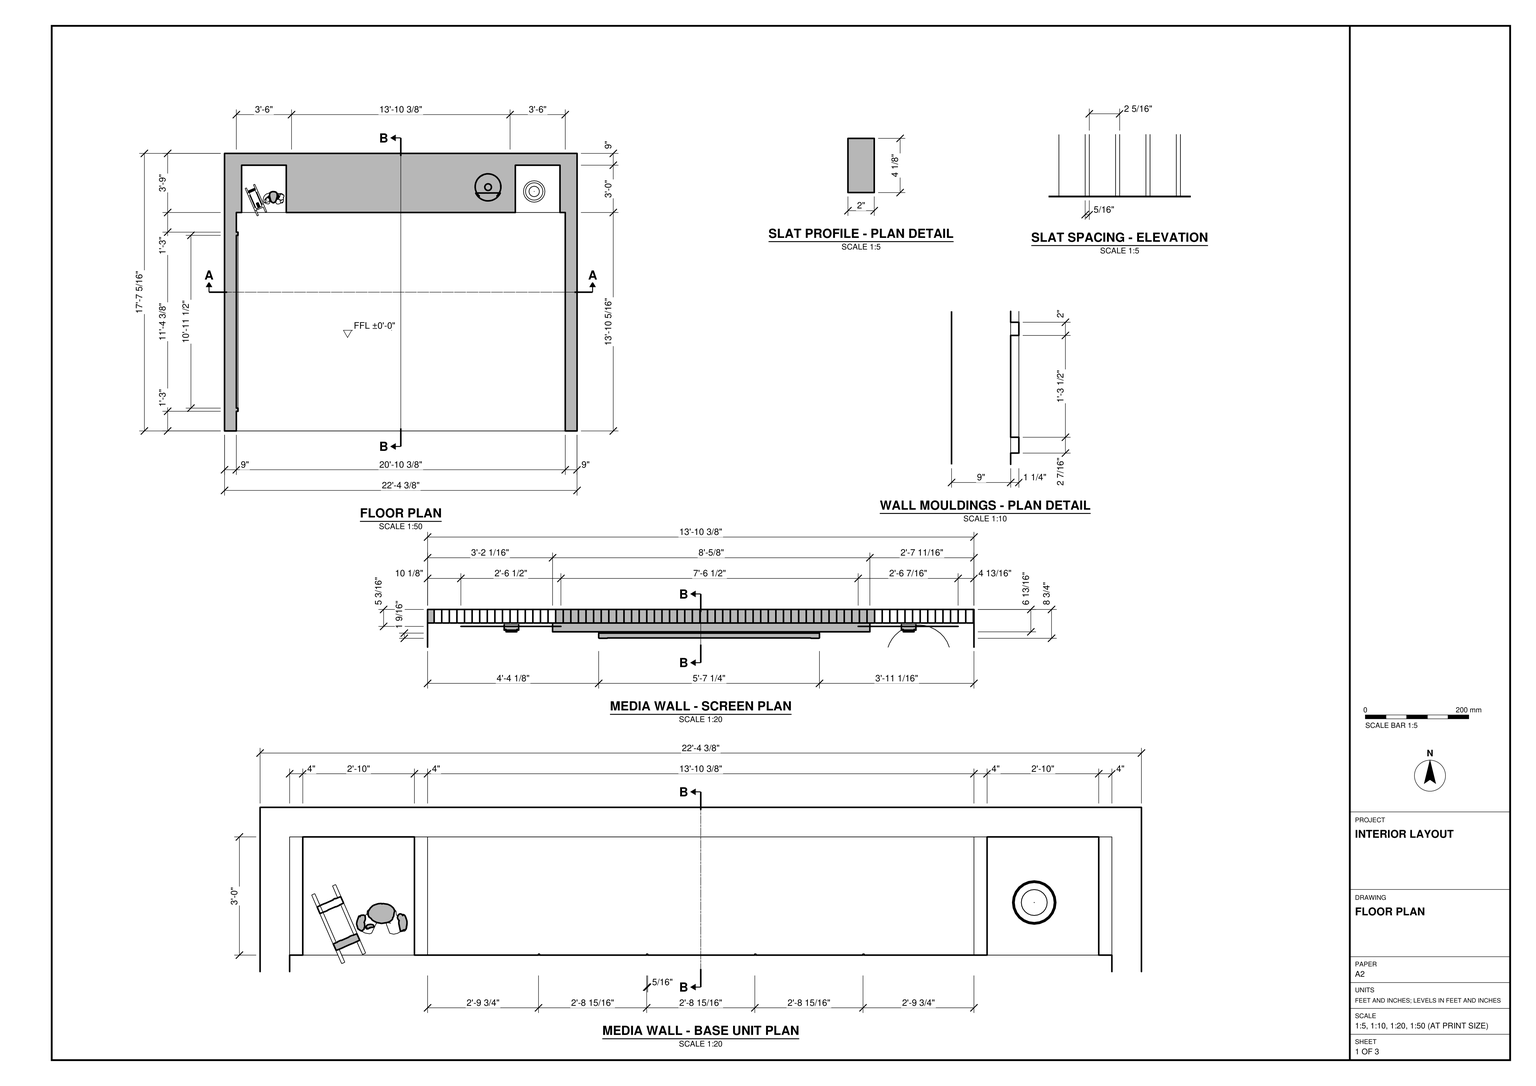
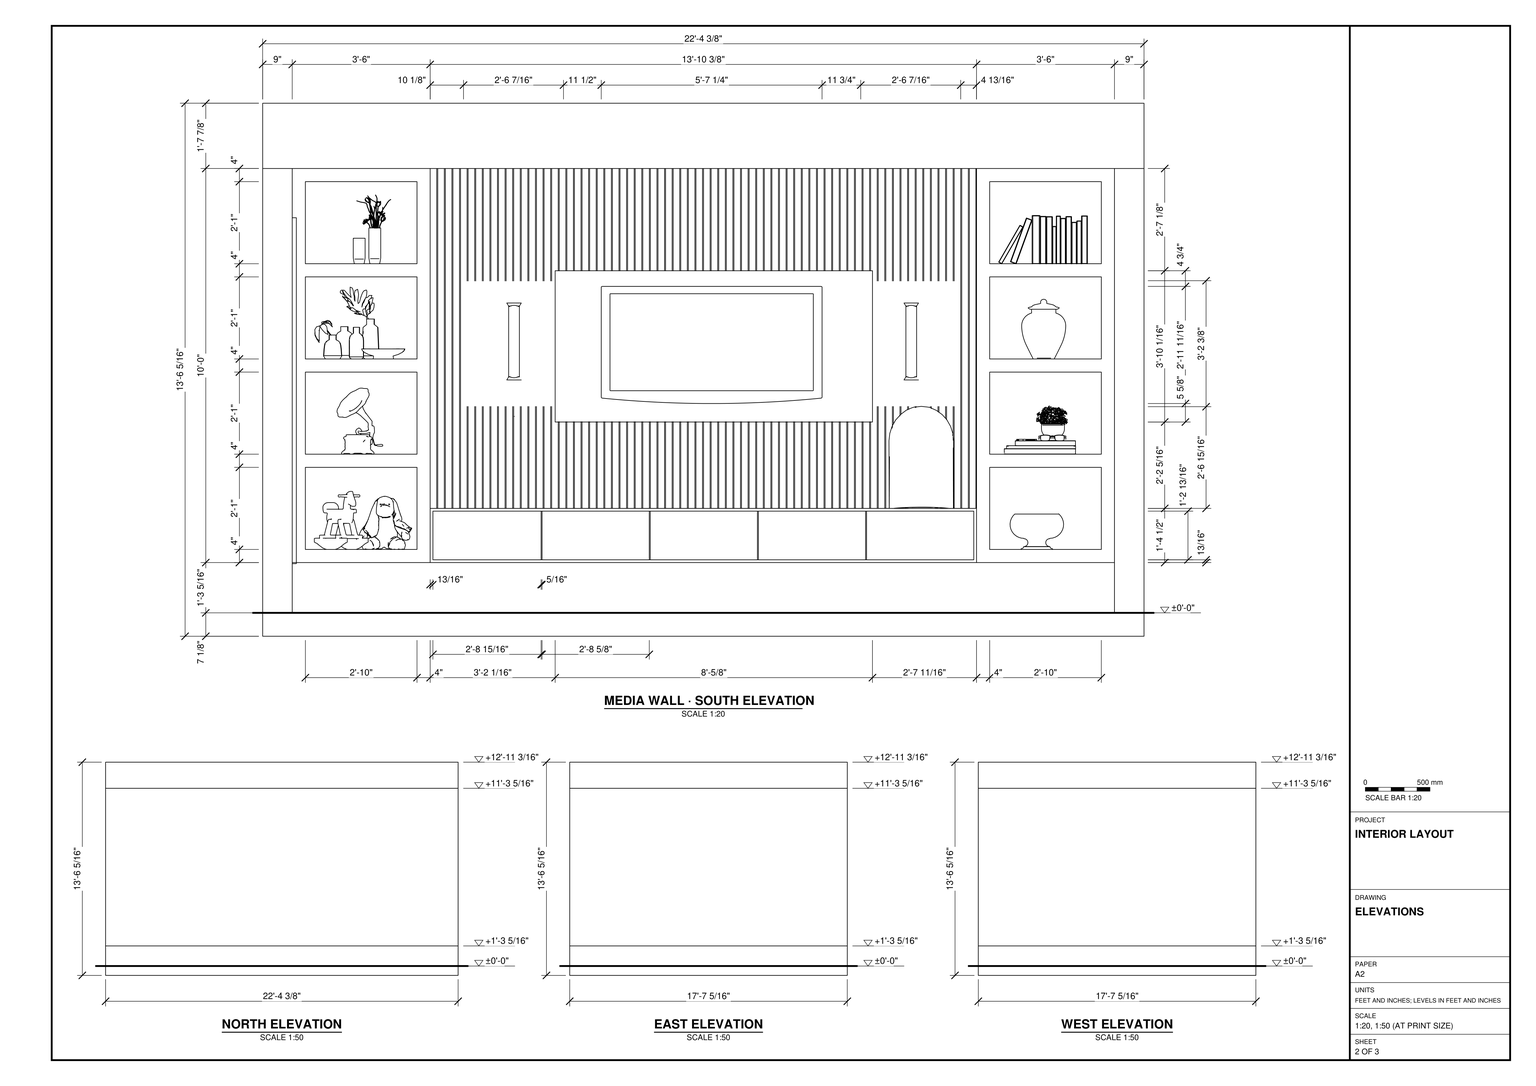
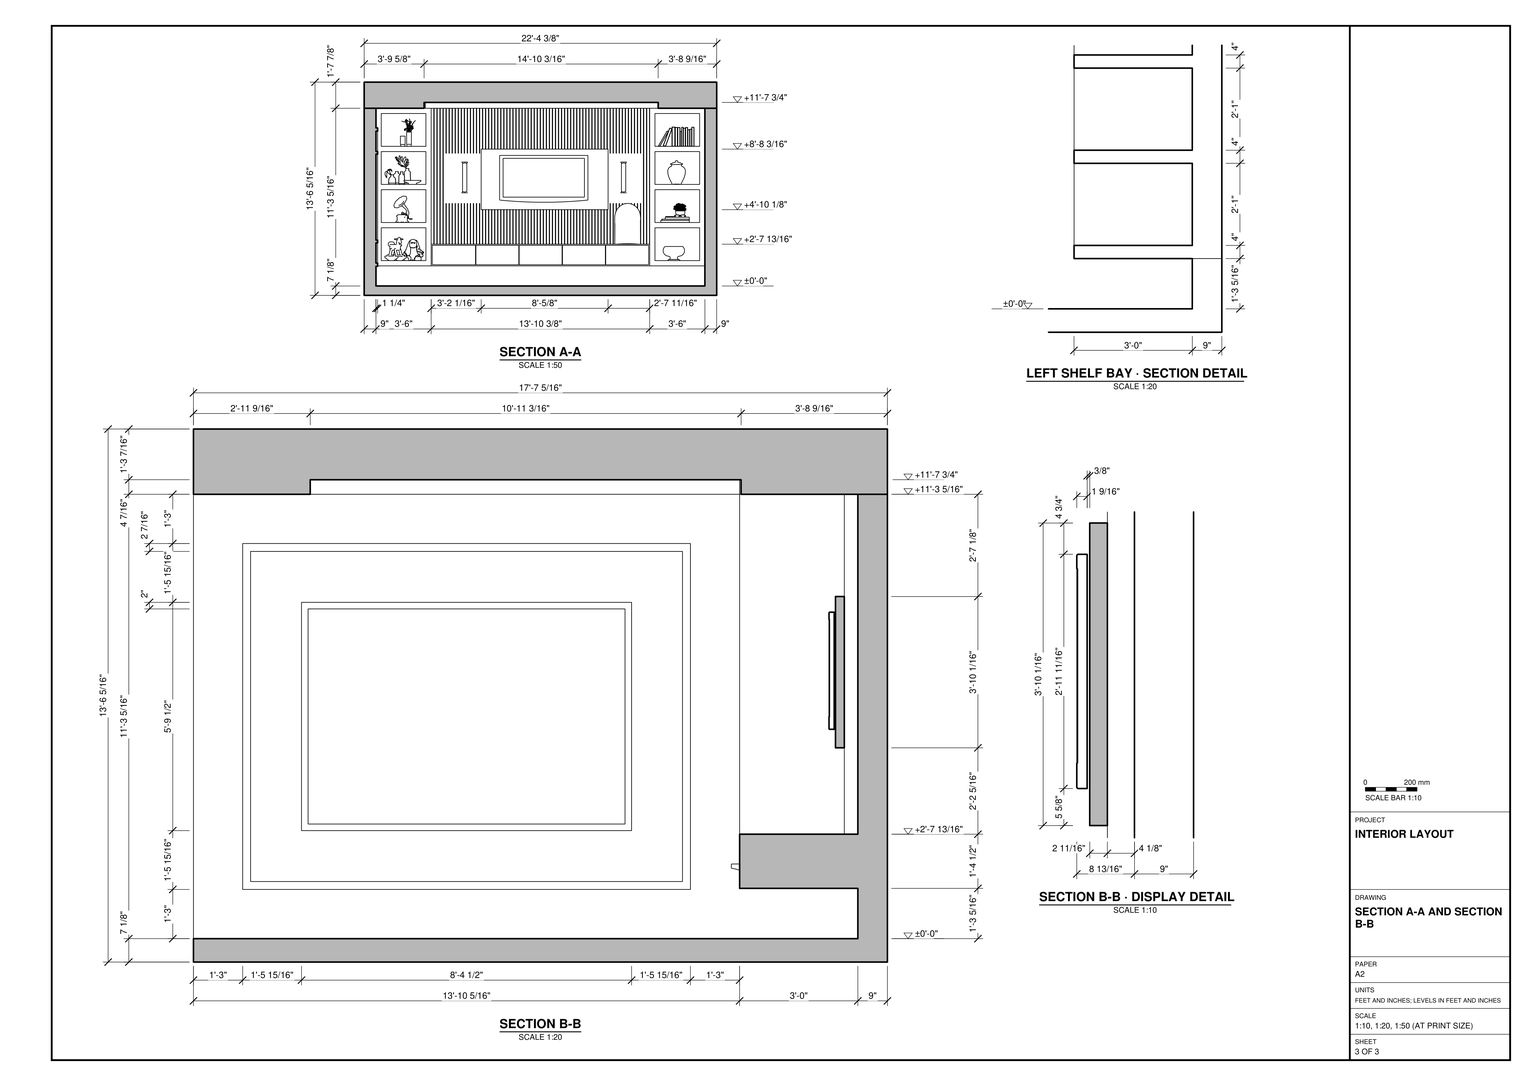
Build the room in SketchUp from task_files/diagram_01.pdf. Work in feet and inches. The overall dimensions are 22'-4 3/8" wide by 17'-7 5/16" deep by 13'-6 5/16" high, with the finished floor at ±0'-0". Follow the plan for the three-sided enclosure, leaving the front open. Model the 9" walls, the floor slab and the ceiling slab. Use the sections to set out the recessed ceiling and the nested rectangular mouldings on the left wall.

Build the media wall across the back of the room. Set out the two shelving bays first, then fit the floating base cabinet and vertical slats between them. Match the five cabinet fronts and align the underside of the cabinet with the underside of the shelf bays. Use the slat profile and spacing detail on sheet 1. Mount the television on its projecting rectangular backing, with a wall light on either side. Follow the elevation for the shelf openings and the placement of books, vessels and other display items. Decor and loose items may be any suitable library components.

Keep the walls, slabs and individual pieces of furniture or joinery in separate groups or components, and use components for repeated parts. Save one SketchUp model as output_files/media_room_with_a_slatted_wall_and_display_shelves.skp.

# SketchUp Ruby script. Lengths in inches.
U = 1.inch
M = Sketchup.active_model
def pt(a) = Geom::Point3d.new(a.map { |v| v * U })
def face(e, loops, mat)
  f = e.add_face(loops[0].map { |a| pt(a) })
  loops[1..].each { |l| e.add_face(l.map { |a| pt(a) }).erase! }
  f.material = f.back_material = mat if mat
  f
end
# faces: each face lists its corners as indices into pts; further lists are holes
def faces(e, pts, list, mat = nil) = list.each { |f| face(e, (f[0].is_a?(Array) ? f : [f]).map { |l| l.map { |i| pts[i] } }, mat) }
# xy, xz, yz: faces in a plane at the given z, y or x. An outline is a flat list of corners, or four numbers for a rectangle; further outlines are holes
def ring(l) = l.size == 4 ? [[l[0], l[1]], [l[2], l[1]], [l[2], l[3]], [l[0], l[3]]] : l.each_slice(2).to_a
def flat(e, list, mat, &to3) = list.each { |f| face(e, (f[0].is_a?(Array) ? f : [f]).map { |l| ring(l).map { |u, v| to3.(u, v) } }, mat) }
def xy(e, z, list, mat = nil) = flat(e, list, mat) { |x, y| [x, y, z] }
def xz(e, y, list, mat = nil) = flat(e, list, mat) { |x, z| [x, y, z] }
def yz(e, x, list, mat = nil) = flat(e, list, mat) { |y, z| [x, y, z] }
def lines(e, pts, list) = list.each { |a, b| e.add_line(pt(pts[a]), pt(pts[b])) }
# prism: a flat outline (further loops are holes) pulled along v
def prism(e, loops, v, mat = nil)
  f = face(e, loops, mat); d = Geom::Vector3d.new(v.map { |x| x * U })
  f.pushpull(f.normal.samedirection?(d) ? d.length : -d.length)
end
def box(e, o, s, mat = nil) = prism(e, [[o, [o[0] + s[0], o[1], o[2]], [o[0] + s[0], o[1] + s[1], o[2]], [o[0], o[1] + s[1], o[2]]]], [0, 0, s[2]], mat)
def at(x, y, z, deg = 0) = Geom::Transformation.translation(pt([x, y, z])) * Geom::Transformation.rotation(ORIGIN, Z_AXIS, deg.degrees)
def axes(o, x, y, z) = Geom::Transformation.new([*x, 0, *y, 0, *z, 0, *pt(o).to_a, 1])
def part(name) = M.definitions.add(name)
# library, detail: a bought-in or finely detailed component or shape, given as its bounding box
def library(name, o, s) = part(name).tap { |d| box(d.entities, o, s) }
def detail(e, o, s) = box(e.add_group.entities, o, s)
def put(e, d, t, mat = nil) = e.add_instance(d, t).tap { |i| i.material = mat if mat }
def group(e, t, mat = nil) = e.add_group.tap { |g| g.transformation = t; g.material = mat if mat }.entities
root = M.entities
M.materials.add("116-1гаусс").color = [249, 237, 214]
M.materials.add("Generic").color = [194, 185, 160]
M.materials.add("Generic\#1").color = [213, 185, 161]
M.materials.add("Generic\#2").color = [232, 206, 193]
M.materials.add("Generic\#3").color = [55, 53, 53]
M.materials.add("Generic\#4").color = [249, 242, 242]
M.materials.add("Generic\#5").color = [215, 202, 161]
M.materials.add("[0027_PeachPuff]").color = [255, 218, 185]
M.materials.add("[Color_000]").color = [255, 255, 255]
M.materials.add("[Color_002]").color = [198, 198, 198]
M.materials.add("[Field Square Tile]").color = [255, 237, 201]
M.materials.add("лампа5-").color = [221, 217, 206]
M.materials.add("ф4").color = [142, 143, 139]
c1 = library("Lidded jar",[0,0,0],[13.42,13.42,18.18])
c2 = library("bell jar",[-16.16,0.46,-16],[33.1,47.04,33.11])
c3 = library("Bowl+I",[-14.3,-14.3,0],[28.6,28.6,19.01])
c4 = library("Group145\#1",[5.875,6.46,9.56],[20.8,10.13,11.36])
c5 = library("books",[6.19,-1.3125,-0.22],[15.35,11.9,12.07])
c6 = library("Untitled",[82.71,28.87,-11.8125],[39.77,1.97,25.2])
c7 = library("Baby Bedroom Swing 189 012",[-5,-14.27,-0.07],[10,28.54,22.18])
c8 = library("Decorative Puppy 209 004",[-5.43,-3.24,0],[10.86,6.48,10.94])
c9 = library("Gramophone 194 010",[-11.96,-11.51,-0.03],[26.29,20.83,37.93])
c10 = library("Vases 103-09",[-7.17,-4.68,0],[14.43,9.35,29.62])
c11 = library("Vase Set 001",[-13.7,-8.6,0],[27.44,16.98,21.89])
c12 = part("Group\#1")
xz(c12.entities,0,[[0,0,2,103.5]])
yz(c12.entities,2,[[0,0,4.125,103.5]])
c13 = part("Группа\#1")
xz(c13.entities,0,[[0,0,13.36,7.23]],"116-1гаусс")
c14 = part("Группа\#3")
put(c14.entities,c13,axes([14.4375,0,0],[0,0,1],[0,1,0],[-1,0,0]))
put(c14.entities,c13,axes([0,0,0],[0,0,1],[0,1,0],[1,0,0]))
c15 = part("Группа\#2")
xy(c15.entities,2.28,[[0,0,1.41,1.41,1.41,34.52,0,35.93],[0,0,10.77,0,10.77,35.93,9.36,34.52,9.36,1.41,1.41,1.41],[1.41,34.52,9.36,34.52,10.77,35.93,0,35.93]],"ф4")
xy(c15.entities,2.59,[[2.52,1.41,2.05,1.54,1.41,1.76,1.41,34.11,2.05,34.33,2.7,34.51,2.73,34.52,8.04,34.52,8.07,34.51,8.72,34.33,9.36,34.11,9.36,1.76,8.72,1.54,8.25,1.41]])
xy(c15.entities,2.59,[[0,0,1.41,1.76,1.41,34.11,0,35.93],[0,0,10.77,0,9.36,1.76,8.72,1.54,8.25,1.41,8.07,1.36,7.4,1.22,6.73,1.12,6.0625,1.05,5.38,1.03,4.71,1.05,4.03,1.12,3.37,1.22,2.7,1.36,2.52,1.41,2.05,1.54,1.41,1.76],[10.77,0,10.77,35.93,9.36,34.11,9.36,1.76],[5.38,1.03,6.0625,1.05,6.73,1.12,7.4,1.22,8.07,1.36,8.25,1.41,2.52,1.41,2.7,1.36,3.37,1.22,4.03,1.12,4.71,1.05],[1.41,34.11,2.05,34.33,2.7,34.51,2.73,34.52,3.37,34.66,4.03,34.76,4.71,34.82,5.38,34.84,6.0625,34.82,6.73,34.76,7.4,34.66,8.04,34.52,8.07,34.51,8.72,34.33,9.36,34.11,10.77,35.93,0,35.93],
  [2.73,34.52,8.04,34.52,7.4,34.66,6.73,34.76,6.0625,34.82,5.38,34.84,4.71,34.82,4.03,34.76,3.37,34.66]],"ф4")
xy(c15.entities,3.36,[[5.38,1.03,6.0625,1.05,6.73,1.12,7.4,1.22,8.07,1.36,8.72,1.54,9.36,1.76,9.36,34.11,8.72,34.33,8.07,34.51,7.4,34.66,6.73,34.76,6.0625,34.82,5.38,34.84,4.71,34.82,4.03,34.76,3.37,34.66,2.7,34.51,2.05,34.33,1.41,34.11,1.41,1.76,2.05,1.54,2.7,1.36,3.37,1.22,4.03,1.12,4.71,1.05]],"лампа5-")
xz(c15.entities,0,[[0,0,10.77,2.28]],"[Color_002]")
xz(c15.entities,0,[[0,2.28,10.77,2.59]],"ф4")
xz(c15.entities,35.93,[[0,0,10.77,2.28]],"[Color_002]")
xz(c15.entities,35.93,[[0,2.28,10.77,2.59]],"ф4")
yz(c15.entities,0,[[0,0,35.93,2.28]],"[Color_002]")
yz(c15.entities,0,[[0,2.28,35.93,2.59]],"ф4")
yz(c15.entities,1.41,[[1.76,2.59,34.11,3.36]])
yz(c15.entities,9.36,[[1.76,2.59,34.11,3.36]],"лампа5-")
yz(c15.entities,10.77,[[0,0,35.93,2.28]],"[Color_002]")
yz(c15.entities,10.77,[[0,2.28,35.93,2.59]],"ф4")
p = [[1.41,1.41,2.28],[0,0,2.28],[0,0,2.59],[1.41,1.41,2.59],[1.41,34.52,2.28],[0,35.93,2.28],
  [0,35.93,2.59],[1.41,34.52,2.59],[10.77,35.93,2.28],[9.36,34.52,2.28],[9.36,34.52,2.59],[10.77,35.93,2.59],
  [5.38,1.03,3.36],[4.71,1.05,3.36],[4.71,1.05,2.59],[5.38,1.03,2.59],[6.0625,1.05,3.36],[6.0625,1.05,2.59],
  [4.03,1.12,3.36],[3.37,1.22,3.36],[3.37,1.22,2.59],[4.03,1.12,2.59],[6.73,1.12,3.36],[6.73,1.12,2.59],
  [7.4,1.22,3.36],[7.4,1.22,2.59],[2.7,1.36,3.36],[2.7,1.36,2.59],[8.07,1.36,3.36],[8.07,1.36,2.59],
  [2.05,1.54,3.36],[2.05,1.54,2.59],[2.52,1.41,2.59],[8.72,1.54,3.36],[8.25,1.41,2.59],[8.72,1.54,2.59],
  [1.41,1.76,3.36],[1.41,1.76,2.59],[9.36,1.76,3.36],[9.36,1.76,2.59],[1.41,34.11,3.36],[2.05,34.33,3.36],
  [2.05,34.33,2.59],[1.41,34.11,2.59],[8.72,34.33,3.36],[9.36,34.11,3.36],[9.36,34.11,2.59],[8.72,34.33,2.59],
  [2.7,34.51,3.36],[2.7,34.51,2.59],[8.07,34.51,3.36],[8.07,34.51,2.59],[3.37,34.66,3.36],[3.37,34.66,2.59],
  [2.73,34.52,2.59],[7.4,34.66,3.36],[8.04,34.52,2.59],[7.4,34.66,2.59],[4.03,34.76,3.36],[4.03,34.76,2.59],
  [6.73,34.76,3.36],[6.73,34.76,2.59],[4.71,34.82,3.36],[4.71,34.82,2.59],[5.38,34.84,3.36],[5.38,34.84,2.59],
  [6.0625,34.82,3.36],[6.0625,34.82,2.59],[9.36,1.41,2.28],[9.36,1.41,2.59]]
faces(c15.entities,p,[[0,1,2,3],[4,5,6,7],[8,9,10,11]],"ф4")
faces(c15.entities,p,[[12,13,14,15],[16,12,15,17],[18,19,20,21],[13,18,21,14],[22,16,17,23],[24,22,23,25],[19,26,27,20],[28,24,25,29],
  [26,30,31,32,27],[33,28,29,34,35],[30,36,37,31],[38,33,35,39]],"лампа5-")
faces(c15.entities,p,[[40,41,42,43],[44,45,46,47],[41,48,49,42],[50,44,47,51],[48,52,53,54,49],[55,50,51,56,57],[52,58,59,53],[60,55,57,61],
  [58,62,63,59],[62,64,65,63],[64,66,67,65],[66,60,61,67]],"[Color_000]")
lines(c15.entities,p,[[68,69]])
c16 = part("Group\#8")
p = [[8.95,0.63,0],[8.88,0.63,0]]
lines(c16.entities,p,[[0,1]])
put(c16.entities,c14,axes([0,0.96,1.71],[1.21923,0,0],[0,1,0],[0,0,1.65953]))
put(c16.entities,c15,axes([7.61,1.27,6.42],[0.23751,0,0],[0,0,0.377],[0,-0.377,0]))
xy(root,-22.4375,[[0,0,268.375,211.3125]])
xy(root,-15.3125,[[9,0,259.375,202.3125]],"[Field Square Tile]")
xy(root,-0.33,[[9,14.98,10.25,151.33]],"Generic\#4")
xy(root,0,[[51,166.3125,217.375,202.3125]],"Generic\#5")
xy(root,0,[[9,166.3125,51,202.3125],[217.375,166.3125,259.375,202.3125]],"[0027_PeachPuff]")
xy(root,0.84,[[84.78,166.3125,85.08,166.61],[117.72,166.3125,118.02,166.61],[150.66,166.3125,150.96,166.61],[183.59,166.3125,183.89,166.61]])
xy(root,2.08,[[9,17.4,10.25,148.92]],"Generic\#4")
xy(root,4,[[13,166.3125,47,202.3125],[221.375,166.3125,255.375,202.3125]],"[0027_PeachPuff]")
xy(root,15.66,[[84.78,166.3125,85.08,166.61],[117.72,166.3125,118.02,166.61],[150.66,166.3125,150.96,166.61],[183.59,166.3125,183.89,166.61]])
xy(root,16.5,[[51,198.1875,53,202.3125]])
xy(root,16.5,[[51,166.3125,217.375,166.3125,217.375,202.3125,53,202.3125,53,198.1875,51,198.1875]],"Generic\#5")
xy(root,17.59,[[9,32.9,10.25,133.41]],"Generic\#4")
xy(root,19.59,[[9,34.9,10.25,131.41]],"Generic\#4")
xy(root,29,[[13,166.3125,47,202.3125],[221.375,166.3125,255.375,202.3125]],"[0027_PeachPuff]")
xy(root,33,[[13,166.3125,47,202.3125],[221.375,166.3125,255.375,202.3125]],"[0027_PeachPuff]")
xy(root,42.8,[[89.0625,195.5,185.6875,198.1875]],"Generic\#5")
xy(root,58,[[13,166.3125,47,202.3125],[221.375,166.3125,255.375,202.3125]],"[0027_PeachPuff]")
xy(root,62,[[221.375,166.3125,255.375,202.3125]],"Generic\#2")
xy(root,62,[[13,166.3125,47,202.3125]],"[0027_PeachPuff]")
xy(root,85.1,[[9,34.9,10.25,131.41]],"Generic\#4")
xy(root,87,[[13,166.3125,47,202.3125],[221.375,166.3125,255.375,202.3125]],"[0027_PeachPuff]")
xy(root,87.1,[[9,32.9,10.25,133.41]],"Generic\#4")
xy(root,88.87,[[89.0625,195.5,185.6875,198.1875]],"Generic\#5")
xy(root,91,[[221.375,166.3125,255.375,202.3125]])
xy(root,91,[[13,166.3125,47,202.3125]],"[0027_PeachPuff]")
xy(root,102.6,[[9,17.4,10.25,148.92]],"Generic\#4")
xy(root,105.02,[[9,14.98,10.25,151.33]],"Generic\#4")
xy(root,116,[[13,166.3125,47,202.3125],[221.375,166.3125,255.375,202.3125]],"[0027_PeachPuff]")
xy(root,120,[[0,0,0,211.3125,268.375,211.3125,268.375,0,259.375,0,259.375,166.3125,223.82,166.3125,223.82,166.76,217.375,166.76,217.375,202.3125,51,202.3125,51,166.76,46.55,166.76,46.55,166.3125,9,166.3125,9,0],[46.55,166.3125,46.55,166.76,46.56,166.76],[46.55,166.3125,51,166.3125,51,166.76,46.56,166.76],[217.375,166.3125,223.5625,166.76],[223.5625,166.3125,223.82,166.76],
  [51,198.1875,53,202.3125]])
xy(root,120,[[9,0,9,166.3125,46.55,166.3125,44.56,35.56,223.82,35.56,223.82,166.76,223.5625,166.76,223.5625,166.3125,259.375,166.3125,259.375,0]],"Generic\#1")
xy(root,120,[[217.375,166.3125,223.5625,166.3125,223.5625,166.76,51,166.76,51,198.1875,53,198.1875,53,202.3125,217.375,202.3125]],"[0027_PeachPuff]")
xy(root,124.4375,[[44.56,35.56,46.55,166.3125,46.55,166.76,223.5625,166.76,223.5625,166.3125,223.82,166.3125,223.82,35.56]],"Generic\#1")
xy(root,139.875,[[0,0,268.375,211.3125]])
xz(root,0,[[0,-22.4375,268.375,-22.4375,268.375,120,259.375,120,259.375,-15.3125,9,-15.3125,9,120,0,120],[0,120,268.375,139.875]])
xz(root,14.98,[[9,-0.33,10.25,0]])
xz(root,14.98,[[9,0,10.25,105.02]],"Generic\#4")
xz(root,17.4,[[9,2.08,10.25,102.6]])
xz(root,32.9,[[9,17.59,10.25,87.1]],"Generic\#4")
xz(root,34.9,[[9,19.59,10.25,85.1]],"Generic\#4")
xz(root,35.56,[[44.56,120,223.82,124.4375]])
xz(root,131.41,[[9,19.59,10.25,85.1]],"Generic\#4")
xz(root,133.41,[[9,17.59,10.25,87.1]],"Generic\#4")
xz(root,148.92,[[9,2.08,10.25,102.6]],"Generic\#4")
xz(root,151.33,[[9,-0.33,10.25,0]])
xz(root,151.33,[[9,0,10.25,105.02]],"Generic\#4")
xz(root,166.3125,[[223.5625,120,223.82,124.4375]])
xz(root,166.3125,[[[51,0,217.375,16.5],[51.84,0.84,216.53,15.66]]],"Generic")
xz(root,166.3125,[[51.84,0.84,84.78,15.66],[85.08,0.84,117.72,15.66],[118.02,0.84,150.66,15.66],[150.96,0.84,183.59,15.66],[183.89,0.84,216.53,15.66]],"Generic\#2")
xz(root,166.3125,[[[9,0,51,120],[13,91,47,116],[13,62,47,87],[13,33,47,58],[13,4,47,29]],[[217.375,0,259.375,120],[221.375,91,255.375,116],[221.375,62,255.375,87],[221.375,33,255.375,58],[221.375,4,255.375,29]]],"Generic\#3")
xz(root,166.61,[[84.78,0.84,85.08,15.66],[117.72,0.84,118.02,15.66],[150.66,0.84,150.96,15.66],[183.59,0.84,183.89,15.66]],"Generic")
xz(root,166.76,[[46.55,120,223.5625,124.4375]],"Generic\#4")
xz(root,195.5,[[89.0625,42.8,185.6875,88.87]],"Generic\#5")
xz(root,198.1875,[[89.0625,42.8,185.6875,88.87]])
xz(root,202.3125,[[51,16.5,53,120],[53,16.5,217.375,120]])
xz(root,202.3125,[[9,-15.3125,259.375,0],[13,4,47,29],[221.375,4,255.375,29],[13,33,47,58],[221.375,33,255.375,58],
  [13,62,47,87],[221.375,62,255.375,87],[13,91,47,116],[221.375,91,255.375,116]],"Generic")
xz(root,211.3125,[[0,-22.4375,268.375,0],[0,0,268.375,120],[0,120,268.375,139.875]])
yz(root,0,[[0,-22.4375,211.3125,0],[0,0,211.3125,120],[0,120,211.3125,139.875]])
yz(root,9,[[[0,-15.3125,202.3125,-15.3125,202.3125,0,166.3125,0,166.3125,120,0,120],[14.98,-0.33,151.33,105.02]],[[17.4,2.08,148.92,102.6],[32.9,17.59,133.41,87.1]],[34.9,19.59,131.41,85.1]],"Generic")
yz(root,10.25,[[[14.98,-0.33,151.33,105.02],[17.4,2.08,148.92,102.6]],[[32.9,17.59,133.41,87.1],[34.9,19.59,131.41,85.1]]],"Generic\#4")
yz(root,13,[[166.3125,4,202.3125,29],[166.3125,33,202.3125,58],[166.3125,62,202.3125,87],[166.3125,91,202.3125,116]],"[0027_PeachPuff]")
yz(root,46.55,[[166.3125,120,166.76,124.4375]])
yz(root,47,[[166.3125,4,202.3125,29],[166.3125,33,202.3125,58],[166.3125,62,202.3125,87],[166.3125,91,202.3125,116]],"[0027_PeachPuff]")
yz(root,51,[[198.1875,16.5,202.3125,120]])
yz(root,51,[[166.3125,16.5,198.1875,120]],"Generic")
yz(root,84.78,[[166.3125,0.84,166.61,15.66]])
yz(root,85.08,[[166.3125,0.84,166.61,15.66]])
yz(root,89.0625,[[195.5,42.8,198.1875,88.87]],"Generic\#5")
yz(root,117.72,[[166.3125,0.84,166.61,15.66]])
yz(root,118.02,[[166.3125,0.84,166.61,15.66]])
yz(root,150.66,[[166.3125,0.84,166.61,15.66]])
yz(root,150.96,[[166.3125,0.84,166.61,15.66]])
yz(root,183.59,[[166.3125,0.84,166.61,15.66]])
yz(root,183.89,[[166.3125,0.84,166.61,15.66]])
yz(root,185.6875,[[195.5,42.8,198.1875,88.87]],"Generic\#5")
yz(root,217.375,[[166.3125,16.5,202.3125,120]],"Generic")
yz(root,221.375,[[166.3125,4,202.3125,29],[166.3125,33,202.3125,58],[166.3125,62,202.3125,87],[166.3125,91,202.3125,116]],"[0027_PeachPuff]")
yz(root,223.5625,[[166.3125,120,166.76,124.4375]])
yz(root,223.82,[[35.56,120,166.3125,124.4375]],"Generic\#4")
yz(root,255.375,[[166.3125,4,202.3125,29],[166.3125,33,202.3125,58],[166.3125,62,202.3125,87],[166.3125,91,202.3125,116]],"[0027_PeachPuff]")
yz(root,259.375,[[0,-15.3125,0,120,166.3125,120,166.3125,0,202.3125,0,202.3125,-15.3125]],"Generic")
yz(root,268.375,[[0,-22.4375,211.3125,0],[0,0,211.3125,120],[0,120,211.3125,139.875]])
p = [[44.56,35.56,120],[46.55,166.3125,120],[46.55,166.3125,124.4375],[44.56,35.56,124.4375]]
faces(root,p,[[0,1,2,3]],"Generic\#4")
put(root,c1,at(231.11,173.0625,62))
put(root,c2,axes([200.78,186.125,13.46],[0.35154,-0.62589,0.05556],[-0.00031,0.06349,0.7172],[-0.62835,-0.35019,0.03073]))
put(root,c3,axes([235.73,182.34,4],[0.57,0,0],[0,0.57,0],[0,0,0.57]))
put(root,c4,axes([216.47,164.12,78.5],[1.3,0,0],[0,1.3,0],[0,0,1.3]))
put(root,c5,axes([217.05,173.55,33.27],[1.4152,0,0],[0,1.22,0],[0,0,1.22]))
put(root,c6,axes([-36.76,164.66,65.15],[1.69092,0,0],[0,1,0],[0,0,1.4157]))
put(root,c7,axes([23.92,175.77,3.99],[0.73309,0.32028,0],[-0.32028,0.73309,0],[0,0,0.8]))
put(root,c8,axes([37.4,177.49,4],[1.48,0,0],[0,1.48,0],[0,0,1.48]))
put(root,c9,axes([28.98,185.92,33.02],[0.5307,0,0],[0,0.5307,0],[0,0,0.5307]),"Generic\#1")
put(root,c10,axes([33.27,180.37,91],[0.79251,0,0],[0,0.7076,0],[0,0,0.7076]))
put(root,c11,at(29.57,184.28,62))
put(root,c12,at(51,198.1875,16.5),"Generic")
put(root,c12,at(53.3125,198.1875,16.5),"Generic")
put(root,c12,at(55.625,198.1875,16.5),"Generic")
put(root,c12,at(57.9375,198.1875,16.5),"Generic")
put(root,c12,at(60.25,198.1875,16.5),"Generic")
put(root,c12,at(62.5625,198.1875,16.5),"Generic")
put(root,c12,at(64.875,198.1875,16.5),"Generic")
put(root,c12,at(67.1875,198.1875,16.5),"Generic")
put(root,c12,at(69.5,198.1875,16.5),"Generic")
put(root,c12,at(71.8125,198.1875,16.5),"Generic")
put(root,c12,at(74.125,198.1875,16.5),"Generic")
put(root,c12,at(76.4375,198.1875,16.5),"Generic")
put(root,c12,at(78.75,198.1875,16.5),"Generic")
put(root,c12,at(81.0625,198.1875,16.5),"Generic")
put(root,c12,at(83.375,198.1875,16.5),"Generic")
put(root,c12,at(85.6875,198.1875,16.5),"Generic")
put(root,c12,at(88,198.1875,16.5),"Generic")
put(root,c12,at(90.3125,198.1875,16.5),"Generic")
put(root,c12,at(92.625,198.1875,16.5),"Generic")
put(root,c12,at(94.9375,198.1875,16.5),"Generic")
put(root,c12,at(97.25,198.1875,16.5),"Generic")
put(root,c12,at(99.5625,198.1875,16.5),"Generic")
put(root,c12,at(101.875,198.1875,16.5),"Generic")
put(root,c12,at(104.1875,198.1875,16.5),"Generic")
put(root,c12,at(106.5,198.1875,16.5),"Generic")
put(root,c12,at(108.8125,198.1875,16.5),"Generic")
put(root,c12,at(111.125,198.1875,16.5),"Generic")
put(root,c12,at(113.4375,198.1875,16.5),"Generic")
put(root,c12,at(115.75,198.1875,16.5),"Generic")
put(root,c12,at(118.0625,198.1875,16.5),"Generic")
put(root,c12,at(120.375,198.1875,16.5),"Generic")
put(root,c12,at(122.6875,198.1875,16.5),"Generic")
put(root,c12,at(125,198.1875,16.5),"Generic")
put(root,c12,at(127.3125,198.1875,16.5),"Generic")
put(root,c12,at(129.625,198.1875,16.5),"Generic")
put(root,c12,at(131.9375,198.1875,16.5),"Generic")
put(root,c12,at(134.25,198.1875,16.5),"Generic")
put(root,c12,at(136.5625,198.1875,16.5),"Generic")
put(root,c12,at(138.875,198.1875,16.5),"Generic")
put(root,c12,at(141.1875,198.1875,16.5),"Generic")
put(root,c12,at(143.5,198.1875,16.5),"Generic")
put(root,c12,at(145.8125,198.1875,16.5),"Generic")
put(root,c12,at(148.125,198.1875,16.5),"Generic")
put(root,c12,at(150.4375,198.1875,16.5),"Generic")
put(root,c12,at(152.75,198.1875,16.5),"Generic")
put(root,c12,at(155.0625,198.1875,16.5),"Generic")
put(root,c12,at(157.375,198.1875,16.5),"Generic")
put(root,c12,at(159.6875,198.1875,16.5),"Generic")
put(root,c12,at(162,198.1875,16.5),"Generic")
put(root,c12,at(164.3125,198.1875,16.5),"Generic")
put(root,c12,at(166.625,198.1875,16.5),"Generic")
put(root,c12,at(168.9375,198.1875,16.5),"Generic")
put(root,c12,at(171.25,198.1875,16.5),"Generic")
put(root,c12,at(173.5625,198.1875,16.5),"Generic")
put(root,c12,at(175.875,198.1875,16.5),"Generic")
put(root,c12,at(178.1875,198.1875,16.5),"Generic")
put(root,c12,at(180.5,198.1875,16.5),"Generic")
put(root,c12,at(182.8125,198.1875,16.5),"Generic")
put(root,c12,at(185.125,198.1875,16.5),"Generic")
put(root,c12,at(187.4375,198.1875,16.5),"Generic")
put(root,c12,at(189.75,198.1875,16.5),"Generic")
put(root,c12,at(192.0625,198.1875,16.5),"Generic")
put(root,c12,at(194.375,198.1875,16.5),"Generic")
put(root,c12,at(196.6875,198.1875,16.5),"Generic")
put(root,c12,at(199,198.1875,16.5),"Generic")
put(root,c12,at(201.3125,198.1875,16.5),"Generic")
put(root,c12,at(203.625,198.1875,16.5),"Generic")
put(root,c12,at(205.9375,198.1875,16.5),"Generic")
put(root,c12,at(208.25,198.1875,16.5),"Generic")
put(root,c12,at(210.5625,198.1875,16.5),"Generic")
put(root,c12,at(212.875,198.1875,16.5),"Generic")
put(root,c12,at(215.1875,198.1875,16.5),"Generic")
put(root,c12,at(217.5,198.1875,16.5))
put(root,c12,at(256.8125,198.1875,16.5))
put(root,c12,at(259.125,198.1875,16.5))
put(root,c16,axes([61.16,195.5,44.51],[1.73,0,0],[0,1.73,0],[0,0,1.73]))
put(root,c16,axes([182.11,195.5,44.51],[1.73,0,0],[0,1.73,0],[0,0,1.73]),"Generic\#5")
